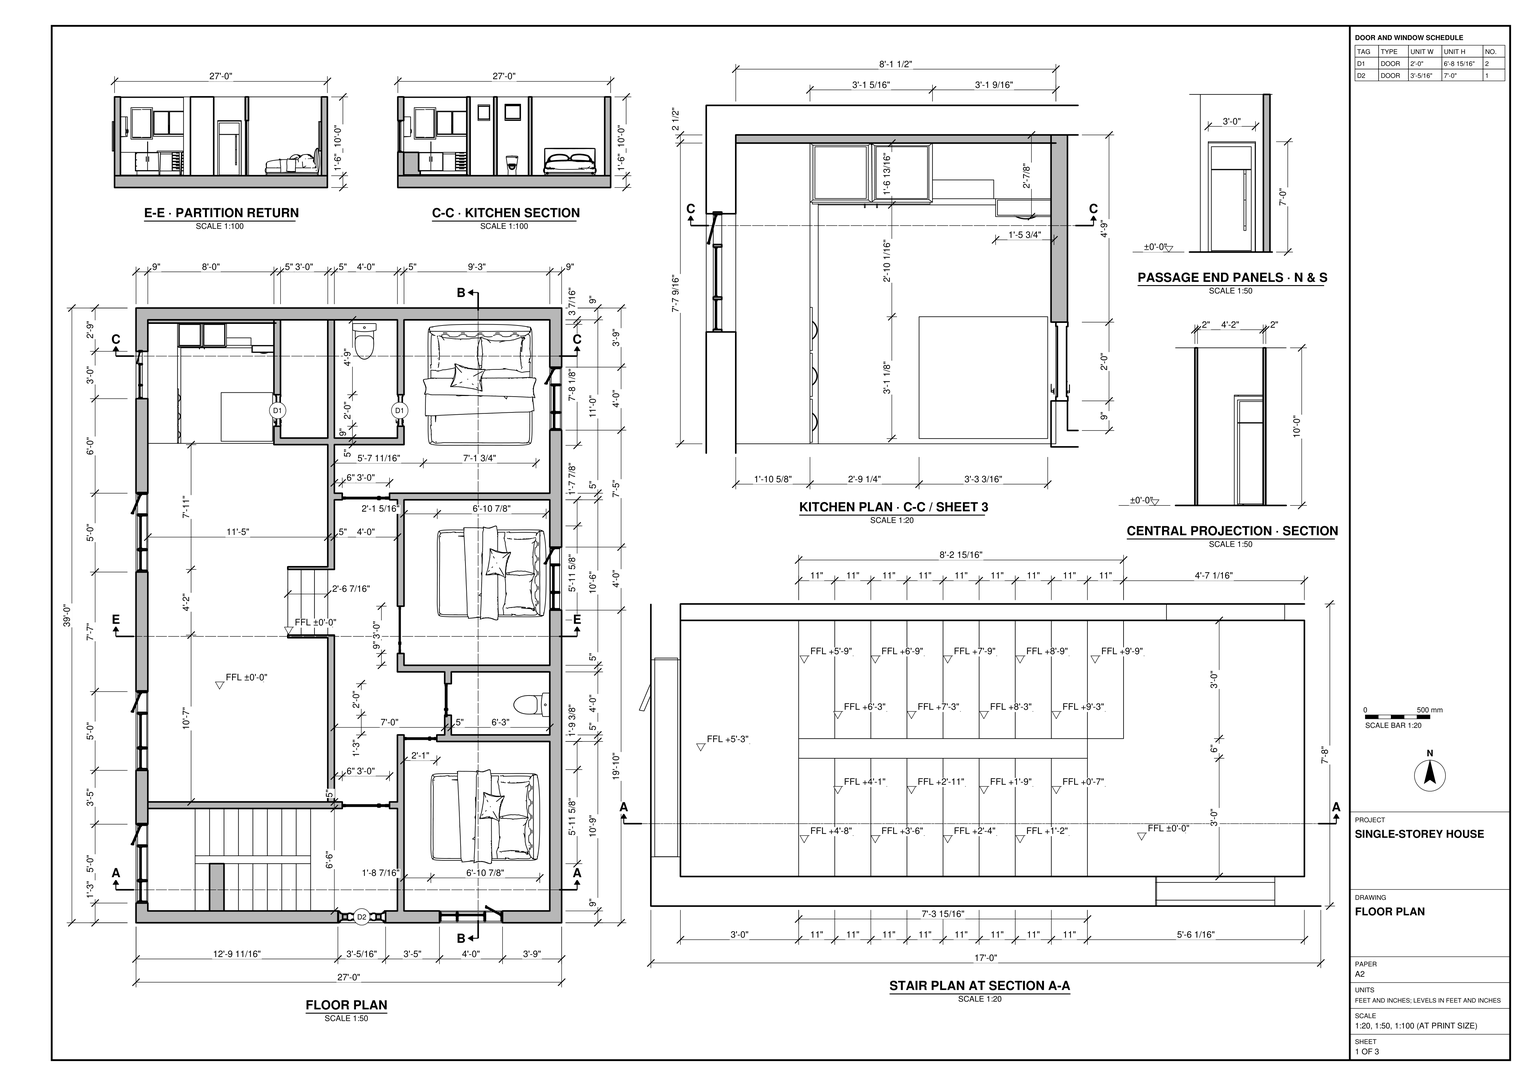
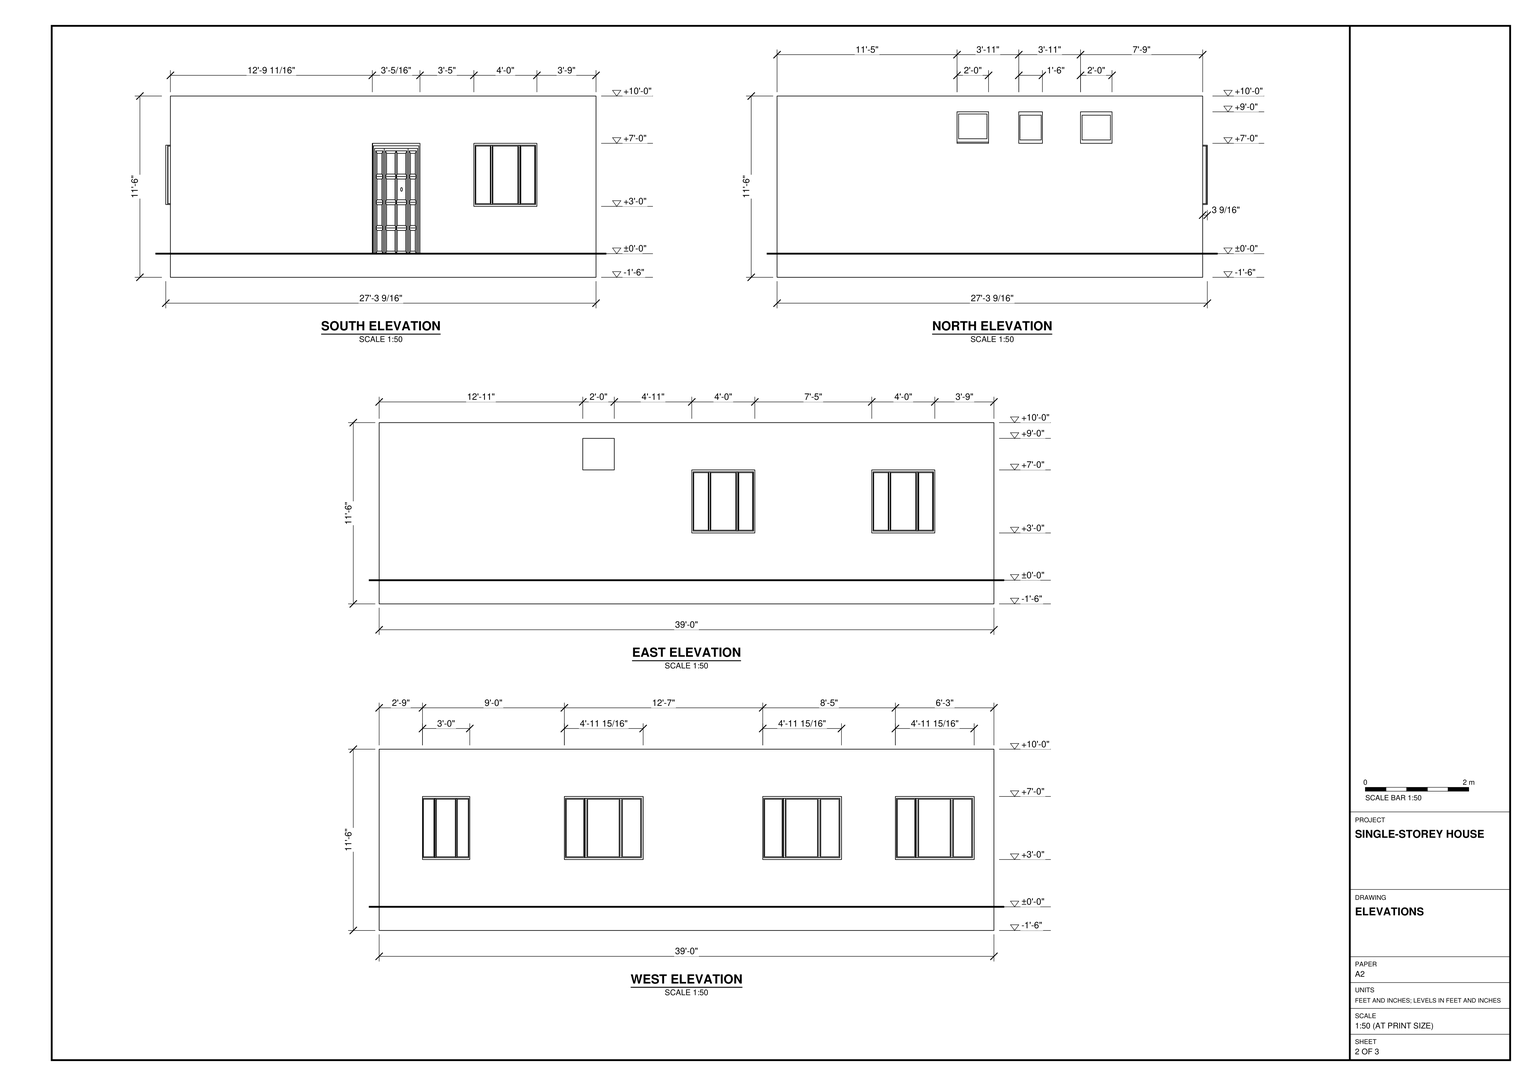
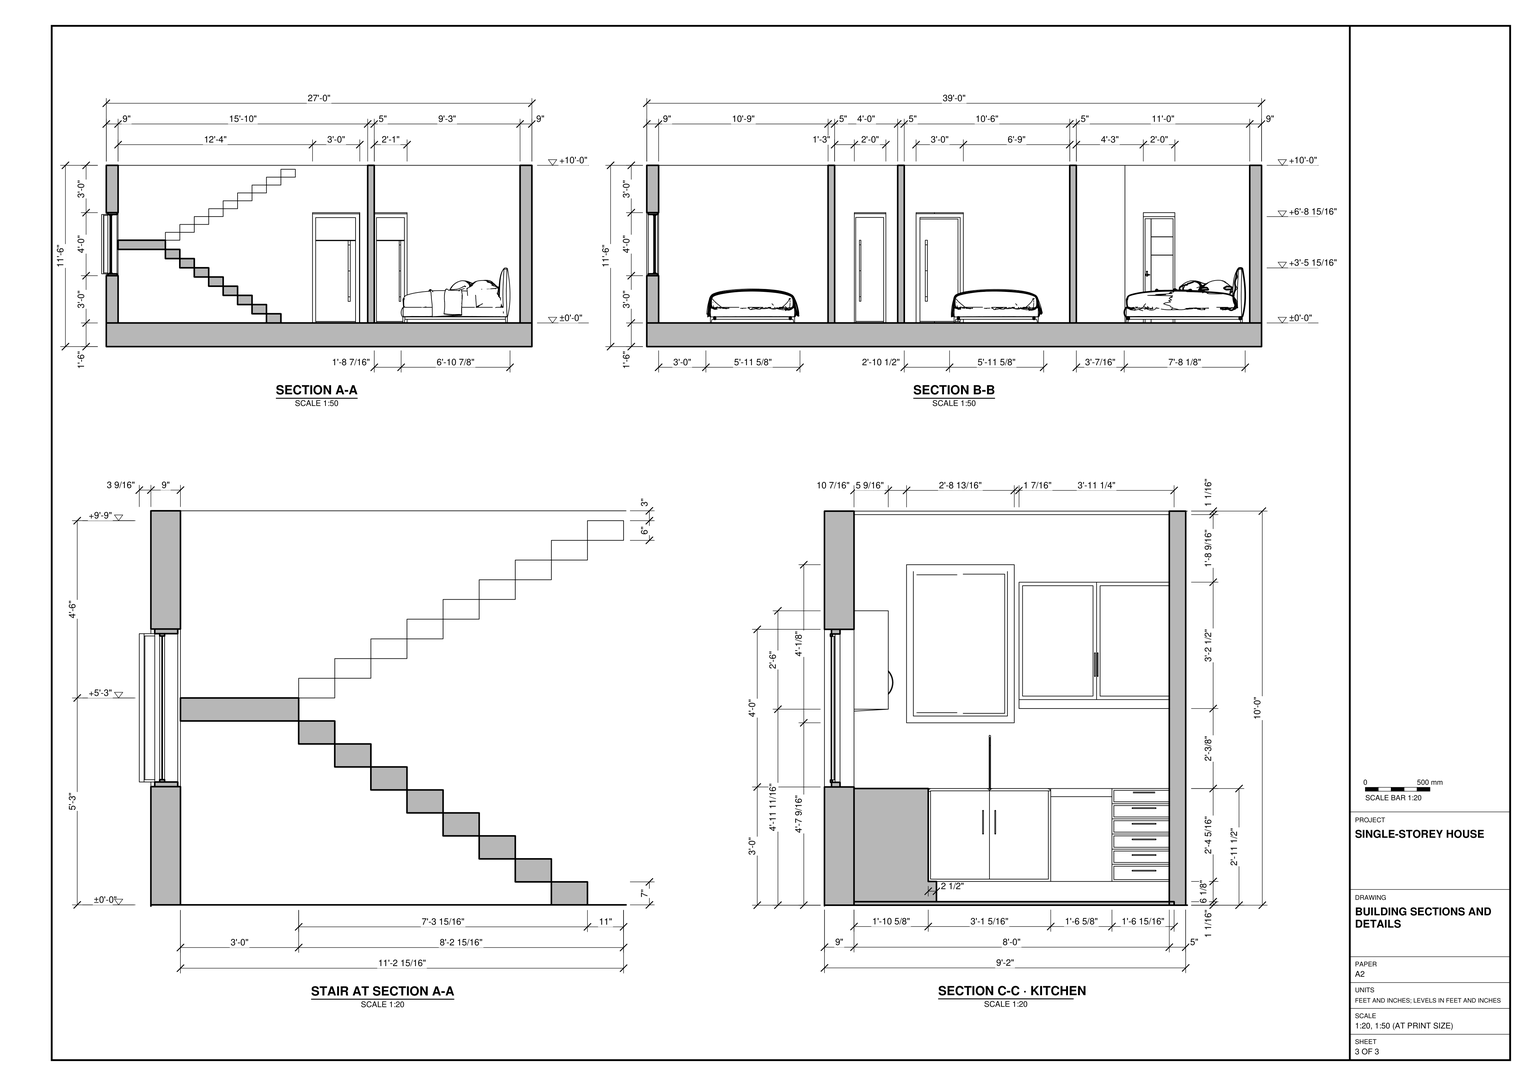
Build the single-storey house in SketchUp from task_files/diagram_01.pdf. Work in feet and inches, with the finished ground floor at ±0'-0". The overall model is 27'-3 9/16" east to west, 39'-0" north to south and 11'-6" high. The rectangular shell itself is 27'-0" wide; use the elevations to account for the projecting window frames rather than widening the walls.

Model the 1'-6" base slab, 9" exterior walls and 5" interior partitions as drawn. Place the entrance on the south side between the stair and the southeast bedroom. Follow the plan for the large open area on the west, the projecting partition return, the three bedrooms along the east side and the two toilet compartments. Fit the doors and window units to the openings shown in the plan and elevations.

Use the enlarged stair plan and section to build the two parallel flights with their shared landing against the west wall. In the northwest kitchen, follow the detailed plan and section for the worktop, base cupboards, drawer bank and wall cupboards. Size and orient the beds from the plan and building sections. Decor and loose items may be any suitable library components.

Keep shell elements separate from one another, make each furniture or joinery piece a separate group or component, and use components for repeated parts. Save one SketchUp model as output_files/single_storey_house_with_return_stair_and_kitchen.skp.

# SketchUp Ruby script. Lengths in inches.
U = 1.inch
M = Sketchup.active_model
def pt(a) = Geom::Point3d.new(a.map { |v| v * U })
def face(e, loops, mat)
  f = e.add_face(loops[0].map { |a| pt(a) })
  loops[1..].each { |l| e.add_face(l.map { |a| pt(a) }).erase! }
  f.material = f.back_material = mat if mat
  f
end
# faces: each face lists its corners as indices into pts; further lists are holes
def faces(e, pts, list, mat = nil) = list.each { |f| face(e, (f[0].is_a?(Array) ? f : [f]).map { |l| l.map { |i| pts[i] } }, mat) }
# xy, xz, yz: faces in a plane at the given z, y or x. An outline is a flat list of corners, or four numbers for a rectangle; further outlines are holes
def ring(l) = l.size == 4 ? [[l[0], l[1]], [l[2], l[1]], [l[2], l[3]], [l[0], l[3]]] : l.each_slice(2).to_a
def flat(e, list, mat, &to3) = list.each { |f| face(e, (f[0].is_a?(Array) ? f : [f]).map { |l| ring(l).map { |u, v| to3.(u, v) } }, mat) }
def xy(e, z, list, mat = nil) = flat(e, list, mat) { |x, y| [x, y, z] }
def xz(e, y, list, mat = nil) = flat(e, list, mat) { |x, z| [x, y, z] }
def yz(e, x, list, mat = nil) = flat(e, list, mat) { |y, z| [x, y, z] }
def lines(e, pts, list) = list.each { |a, b| e.add_line(pt(pts[a]), pt(pts[b])) }
# prism: a flat outline (further loops are holes) pulled along v
def prism(e, loops, v, mat = nil)
  f = face(e, loops, mat); d = Geom::Vector3d.new(v.map { |x| x * U })
  f.pushpull(f.normal.samedirection?(d) ? d.length : -d.length)
end
def box(e, o, s, mat = nil) = prism(e, [[o, [o[0] + s[0], o[1], o[2]], [o[0] + s[0], o[1] + s[1], o[2]], [o[0], o[1] + s[1], o[2]]]], [0, 0, s[2]], mat)
def at(x, y, z, deg = 0) = Geom::Transformation.translation(pt([x, y, z])) * Geom::Transformation.rotation(ORIGIN, Z_AXIS, deg.degrees)
def axes(o, x, y, z) = Geom::Transformation.new([*x, 0, *y, 0, *z, 0, *pt(o).to_a, 1])
def part(name) = M.definitions.add(name)
# library, detail: a bought-in or finely detailed component or shape, given as its bounding box
def library(name, o, s) = part(name).tap { |d| box(d.entities, o, s) }
def detail(e, o, s) = box(e.add_group.entities, o, s)
def put(e, d, t, mat = nil) = e.add_instance(d, t).tap { |i| i.material = mat if mat }
def group(e, t, mat = nil) = e.add_group.tap { |g| g.transformation = t; g.material = mat if mat }.entities
root = M.entities
M.materials.add("Doors_Windows").color = [200, 200, 200]
M.materials.add("Rectangles Running 2x1").color = [231, 231, 231]
M.materials.add("[0011_Seashell]").color = [255, 245, 238]
M.materials.add("[0130_Gainsboro]").color = [220, 220, 220]
M.materials.add("[Color_000]").color = [255, 255, 255]
M.materials.add("[Metal_Aluminum_Anodized]1").color = [202, 209, 219]
M.materials.add("[Stone_Masonry_Multi]").color = [182, 175, 164]
M.materials.add("[Stone_Sandstone_Ashlar_Light]1").color = [206, 178, 128]
M.materials.add("[Translucent Glass Blue]").color = [100, 149, 237]
M.materials["[Translucent Glass Blue]"].alpha = 0.5
M.materials.add("[Translucent_Glass_Safety]").color = [204, 235, 244]
M.materials["[Translucent_Glass_Safety]"].alpha = 0.5
M.materials.add("[Wood Cherry Original]").color = [152, 86, 42]
M.materials.add("[Wood_Bamboo_Medium]").color = [177, 105, 43]
M.materials.add("[Wood_Floor_Parquet]").color = [145, 89, 39]
M.materials.add("[Wood_OSB]").color = [240, 195, 122]
c1 = part("bod vindu")
g1 = group(c1.entities,at(0,-46.85,0),"[Translucent Glass Blue]")
yz(g1,0.94,[[2.36,2.36,44.49,19.65]],"[Translucent Glass Blue]")
# 2 loose lines left out
g2 = group(g1,at(0,46.85,0,-90),"[Color_000]")
xy(g2,0,[[0,0,46.85,3.9375]])
xy(g2,1.57,[[1.57,0,45.28,0.55]])
xy(g2,2.36,[[2.36,0.55,44.49,3.9375]])
xy(g2,19.65,[[2.36,0.55,4.29,3.9375],[4.29,0.55,44.49,3.9375]])
xy(g2,20.43,[[1.57,0,45.28,0.55]])
xy(g2,22.01,[[0,0,46.85,3.9375]])
xz(g2,0,[[[0,0,46.85,22.01],[1.57,1.57,45.28,20.43]]])
xz(g2,0.55,[[1.57,1.57,45.28,2.36],[1.57,2.36,2.36,2.36,2.36,19.65,44.49,19.65,44.49,2.36,45.28,2.36,45.28,20.43,1.57,20.43]])
xz(g2,3.9375,[[[0,0,46.85,22.01],[2.36,2.36,44.49,19.65]]])
yz(g2,0,[[0,0,3.9375,22.01]])
yz(g2,1.57,[[0,1.57,0.55,2.36,0.55,20.43,0,20.43]])
yz(g2,2.36,[[0.55,2.36,3.9375,19.65]])
yz(g2,44.49,[[0.55,2.36,3.9375,19.65]])
yz(g2,45.28,[[0,1.57,0,20.43,0.55,20.43,0.55,2.36]])
yz(g2,46.85,[[0,0,3.9375,22.01]])
p = [[45.28,0,1.57],[1.57,0,1.57],[1.57,0.55,2.36],[2.36,0.55,2.36],[44.49,0.55,2.36],[45.28,0.55,2.36]]
faces(g2,p,[[0,1,2,3,4,5]])
c2 = library("Door",[0,0,0],[79.98,10,87.99])
c3 = library("porta de madeira",[3.7,-4.82,1.36],[53.55,7.65,83.26])
c4 = library("Door\#1",[0,0,0],[31.5,7.64,86.61])
c5 = library("CS300DRT",[0,0,0],[27.18,17.85,30.31])
c6 = part("Group\#36")
box(c6.entities,[-2,0,0],[2,7,64])
c7 = part("Group\#6")
xy(c7.entities,0,[[0,-7,96,0]])
xy(c7.entities,2,[[2,-7,94,0]])
xy(c7.entities,66,[[2,-7,94,0]])
xy(c7.entities,68,[[0,-7,96,0]])
xz(c7.entities,-7,[[[0,0,96,68],[2,2,94,66]]])
xz(c7.entities,0,[[[0,0,96,68],[2,2,94,66]]])
yz(c7.entities,0,[[-7,0,0,68]])
yz(c7.entities,2,[[-7,2,0,66]])
yz(c7.entities,94,[[-7,2,0,66]])
yz(c7.entities,96,[[-7,0,0,68]])
put(c7.entities,c6,at(70,-7,2))
put(c7.entities,c6,at(28,-7,2))
g3 = group(c7.entities,at(70.82,4.71,2,-15),"[Translucent Glass Blue]")
xy(g3,0,[[0,-1.5,24,0]],"Doors_Windows")
xy(g3,1,[[1,-1.5,23,-0.75],[1,-0.75,23,0]],"Doors_Windows")
xy(g3,63,[[1,-1.5,23,-0.75],[1,-0.75,23,0]],"Doors_Windows")
xy(g3,64,[[0,-1.5,24,0]],"Doors_Windows")
xz(g3,-1.5,[[[0,0,24,64],[1,1,23,63]]],"Doors_Windows")
xz(g3,-0.75,[[1,1,23,63]],"[Translucent Glass Blue]")
xz(g3,0,[[[0,0,24,64],[1,1,23,63]]],"Doors_Windows")
yz(g3,0,[[-1.5,0,0,64]],"Doors_Windows")
yz(g3,1,[[-1.5,1,-0.75,63],[-0.75,1,0,63]],"Doors_Windows")
yz(g3,23,[[-1.5,1,-0.75,63],[-0.75,1,0,63]],"Doors_Windows")
yz(g3,24,[[-1.5,0,0,64]],"Doors_Windows")
g4 = group(c7.entities,at(2,-1.5,2))
xy(g4,0,[[0,-1.5,24,0]],"[Translucent Glass Blue]")
xy(g4,1,[[1,-1.5,23,-0.75],[1,-0.75,23,0]],"[Translucent Glass Blue]")
xy(g4,63,[[1,-1.5,23,-0.75],[1,-0.75,23,0]],"[Translucent Glass Blue]")
xy(g4,64,[[0,-1.5,24,0]],"[Translucent Glass Blue]")
xz(g4,-1.5,[[[0,0,24,64],[1,1,23,63]]],"[Translucent Glass Blue]")
xz(g4,-0.75,[[1,1,23,63]],"[Translucent Glass Blue]")
xz(g4,0,[[[0,0,24,64],[1,1,23,63]]],"[Translucent Glass Blue]")
yz(g4,0,[[-1.5,0,0,64]],"[Translucent Glass Blue]")
yz(g4,1,[[-1.5,1,-0.75,63],[-0.75,1,0,63]],"[Translucent Glass Blue]")
yz(g4,23,[[-1.5,1,-0.75,63],[-0.75,1,0,63]],"[Translucent Glass Blue]")
yz(g4,24,[[-1.5,0,0,64]],"[Translucent Glass Blue]")
g5 = group(c7.entities,at(28,-1.5,2),"[Translucent Glass Blue]")
xy(g5,0,[[0,-1.5,40,0]],"Doors_Windows")
xy(g5,1,[[1,-1.5,39,-0.75],[1,-0.75,39,0]],"Doors_Windows")
xy(g5,63,[[1,-1.5,39,-0.75],[1,-0.75,39,0]],"Doors_Windows")
xy(g5,64,[[0,-1.5,40,0]],"Doors_Windows")
xz(g5,-1.5,[[[0,0,40,64],[1,1,39,63]]],"Doors_Windows")
xz(g5,-0.75,[[1,1,39,63]],"[Translucent Glass Blue]")
xz(g5,0,[[[0,0,40,64],[1,1,39,63]]],"Doors_Windows")
yz(g5,0,[[-1.5,0,0,64]],"Doors_Windows")
yz(g5,1,[[-1.5,1,-0.75,63],[-0.75,1,0,63]],"Doors_Windows")
yz(g5,39,[[-1.5,1,-0.75,63],[-0.75,1,0,63]],"Doors_Windows")
yz(g5,40,[[-1.5,0,0,64]],"Doors_Windows")
c8 = part("Group\#84")
box(c8.entities,[0,0,0],[10.99,36,7])
c9 = part("Group\#85")
box(c9.entities,[0,0,0],[10.99,36,6])
c10 = library("Group10",[-94.75,-3.97,0],[199.87,106.11,39.4375])
c11 = library("mesh-258",[-96.03,-121.28,21.97],[201.42,163.89,40.48])
c12 = library("Group14",[-46.92,-34.29,0],[94.87,68.58,31.875])
c13 = library("Group16",[-47.82,-34.55,0],[96.75,69.58,33.34])
c14 = library("Group18",[-33.62,-26.58,0],[67.24,53.16,20.44])
c15 = library("Group20",[-0.01,-0.01,0.02],[107.76,124.16,6.31])
c16 = library("mesh-263",[-97.08,-118.58,12.75],[201.41,233.93,94.93])
c17 = library("mesh-264",[-106.11,-80.86,12.52],[217.88,74.95,54.44])
c18 = part("Group9")
put(c18.entities,c10,axes([-2.83,3.64,23.125],[0.96274,0,0],[0,0.96274,0],[0,0,0.96274]))
g6 = group(c18.entities,at(-2.83,3.64,23.41))
put(g6,c11,axes([0,0,-21.09],[0.96274,0,0],[0,0.96274,0],[0,0,0.96274]))
put(c18.entities,c12,at(49.15,58.47,50.125))
put(c18.entities,c13,at(-47.3,60.89,49.06))
put(c18.entities,c14,at(-22.74,14.21,61.08))
put(c18.entities,c15,axes([-96.54,-113.26,0],[1.80992,0,0],[0,1.80992,0],[0,0,1.80992]))
g7 = group(c18.entities,at(-2.83,1.61,11.33))
put(g7,c16,at(0,0,-12.75))
g8 = group(c18.entities,at(-2.83,20.36,11.1))
put(g8,c17,at(0,0,-12.52))
c19 = library("Group\#91",[0,0,0],[8.9,40.12,1.52])
c20 = part("Group\#92")
xy(c20.entities,0,[[0,0,117.79,26.26]])
c21 = part("Group\#93")
box(c21.entities,[0,0,0],[32.88,158.35,2.28])
c22 = part("Tapered column")
xy(c22.entities,0,[[0,0,24.46,29.02]])
xy(c22.entities,262.42,[[7.21,8.5625,17.24,20.46]])
p = [[7.21,8.5625,262.42],[7.21,20.46,262.42],[0,29.02,0],[0,0,0],[24.46,0,0],[17.24,8.5625,262.42],
  [24.46,29.02,0],[17.24,20.46,262.42]]
faces(c22.entities,p,[[0,1,2,3],[4,5,0,3],[4,6,7,5],[2,1,7,6]])
xy(root,1.07,[[12.54,364.95,37.64,364.95,37.64,437.69,110.01,437.69,110.01,456.52,12.54,456.52]])
xy(root,7.22,[[35.13,364.95,37.64,438.5],[37.64,437.69,37.64,438.5,72.43,438.5,72.43,439.58,110.01,439.58,110.01,437.69]],"[Wood_Bamboo_Medium]")
xy(root,7.79,[[35.13,365.375,35.85,378.5],[35.13,379.36,35.85,392.49],[35.13,393.35,35.85,406.47],[91.66,439.04,109.43,439.58]])
xy(root,7.93,[[35.85,437.96,37.64,438.5],[37.64,437.96,71.71,438.5]])
xy(root,11.87,[[91.66,439.04,109.43,439.58]],"[Wood_Bamboo_Medium]")
xy(root,13,[[91.66,439.04,109.43,439.58]])
xy(root,16.49,[[35.13,365.375,35.85,378.5],[35.13,379.36,35.85,392.49],[35.13,393.35,35.85,406.47],[91.66,439.04,109.43,439.58]],"[Wood_Bamboo_Medium]")
xy(root,17.62,[[35.13,365.375,35.85,378.5],[35.13,379.36,35.85,392.49],[35.13,393.35,35.85,406.47],[91.66,439.04,109.43,439.58]])
xy(root,21.1,[[91.66,439.04,109.43,439.58]],"[Wood_Bamboo_Medium]")
xy(root,22.24,[[91.66,439.04,109.43,439.58]])
xy(root,25.72,[[35.13,365.375,35.85,378.5],[35.13,379.36,35.85,392.49],[35.13,393.35,35.85,406.47],[91.66,439.04,109.43,439.58]],"[Wood_Bamboo_Medium]")
xy(root,26.86,[[35.13,365.375,35.85,378.5],[35.13,379.36,35.85,392.49],[91.66,439.04,109.43,439.58]])
xy(root,26.86,[[35.13,393.35,35.85,406.47]],"[Wood_Bamboo_Medium]")
xy(root,30.34,[[91.66,439.04,109.43,439.58]],"[Wood_Bamboo_Medium]")
xy(root,31.48,[[91.66,434.12,109.43,439.58]],"[Wood_Bamboo_Medium]")
xy(root,32.6875,[[36.64,439.63,52.28,455.39],[55.29,439.63,70.93,455.39]],"[Metal_Aluminum_Anodized]1")
xy(root,33.06,[[72.43,439.58,91.08,445.3]],"Rectangles Running 2x1")
xy(root,33.24,[[92.23,434.55,108.86,439.15]],"[Wood_Bamboo_Medium]")
xy(root,34.82,[[35.85,437.96,71.71,438.5]],"[Wood_Bamboo_Medium]")
xy(root,34.96,[[35.13,365.375,35.85,378.5],[35.13,379.36,35.85,392.49],[35.13,393.35,35.85,406.47],[[91.66,434.12,109.43,439.58],[92.23,434.55,108.86,439.15]]],"[Wood_Bamboo_Medium]")
xy(root,35.53,[[12.54,364.95,35.13,456.52],[91.08,439.58,110.01,439.58,110.01,456.52,72.43,456.52,72.43,445.3,91.08,445.3]],"Rectangles Running 2x1")
xy(root,35.53,[[[36.03,439.17,52.89,455.85],[36.64,439.63,52.28,455.39]],[[54.87,439.32,71.34,455.7],[55.29,439.63,70.93,455.39]]],"[Metal_Aluminum_Anodized]1")
xy(root,55.54,[[28.53,456.52,61.33,459]],"[0011_Seashell]")
xy(root,59.67,[[12.54,364.95,21.21,380.1],[12.54,380.1,20.03,395.21]],"[0130_Gainsboro]")
xy(root,59.88,[[62.78,450.85,110.01,456.52]],"[Wood_Floor_Parquet]")
xy(root,61.48,[[20.5,364.95,21.21,380.1],[18.13,380.1,20.03,395.21]],"[0130_Gainsboro]")
xy(root,63.67,[[63.86,450.85,85.32,455.72],[87.47,450.85,108.93,455.72]],"[Wood_Floor_Parquet]")
xy(root,65.32,[[12.54,425.35,18.53,425.73]])
xy(root,65.32,[[12.54,404.09,18.53,404.5]],"[Wood_Bamboo_Medium]")
xy(root,74.57,[[63.86,452.14,85.32,455.72]],"[Wood_Floor_Parquet]")
xy(root,84.03,[[12.54,404.09,18.53,404.5]],"[Wood_Bamboo_Medium]")
xy(root,89.65,[[12.54,364.95,20.5,380.1],[12.54,380.1,18.13,395.21],[12.54,432.6,22.97,456.52]],"[0130_Gainsboro]")
xy(root,97.29,[[63.86,450.85,85.32,455.72],[87.47,450.85,108.93,455.72]],"[Wood_Floor_Parquet]")
xy(root,98.35,[[62.78,450.85,110.01,456.52]],"[Wood_Floor_Parquet]")
xy(root,103.68,[[28.53,456.52,61.33,459]],"[0011_Seashell]")
xz(root,364.95,[[12.54,59.67,12.54,89.65,20.5,89.65,20.5,61.48,21.21,61.48,21.21,59.67]],"[0130_Gainsboro]")
xz(root,364.95,[[12.54,1.07,12.54,35.53,35.13,35.53,35.13,7.22,37.64,7.22,37.64,1.07]],"[Wood_Bamboo_Medium]")
xz(root,365.375,[[35.13,7.79,35.85,16.49],[35.13,17.62,35.85,25.72],[35.13,26.86,35.85,34.96]],"[Wood_Bamboo_Medium]")
xz(root,378.5,[[35.13,7.79,35.85,16.49],[35.13,17.62,35.85,25.72],[35.13,26.86,35.85,34.96]],"[Wood_Bamboo_Medium]")
xz(root,379.36,[[35.13,7.79,35.85,16.49],[35.13,17.62,35.85,25.72],[35.13,26.86,35.85,34.96]],"[Wood_Bamboo_Medium]")
xz(root,380.1,[[12.54,59.67,20.03,59.67,20.03,61.48,18.13,61.48,18.13,89.65,12.54,89.65]])
xz(root,380.1,[[20.03,59.67,21.21,59.67,21.21,61.48,20.5,61.48,20.5,89.65,18.13,89.65,18.13,61.48,20.03,61.48]],"[0130_Gainsboro]")
xz(root,392.49,[[35.13,7.79,35.85,16.49],[35.13,17.62,35.85,25.72],[35.13,26.86,35.85,34.96]],"[Wood_Bamboo_Medium]")
xz(root,393.35,[[35.13,7.79,35.85,16.49],[35.13,17.62,35.85,25.72],[35.13,26.86,35.85,34.96]],"[Wood_Bamboo_Medium]")
xz(root,395.21,[[12.54,59.67,20.03,59.67,20.03,61.48,18.13,61.48,18.13,89.65,12.54,89.65]],"[0130_Gainsboro]")
xz(root,404.09,[[12.54,65.32,18.53,84.03]],"[Wood_Bamboo_Medium]")
xz(root,404.5,[[12.54,65.32,18.53,84.03]],"[Wood_Bamboo_Medium]")
xz(root,406.47,[[35.13,7.79,35.85,16.49],[35.13,17.62,35.85,25.72],[35.13,26.86,35.85,34.96]],"[Wood_Bamboo_Medium]")
xz(root,425.35,[[12.54,65.32,18.53,65.32,18.53,84.03,12.54,83.89]],"[Wood_Bamboo_Medium]")
xz(root,425.73,[[12.54,65.32,12.54,83.89,18.53,84.03,18.53,65.32]],"[Wood_Bamboo_Medium]")
xz(root,432.6,[[12.54,59.67,22.97,89.65]],"[0130_Gainsboro]")
xz(root,434.12,[[91.66,31.48,109.43,34.96]],"[Wood_Bamboo_Medium]")
xz(root,434.55,[[92.23,33.24,108.86,34.96]])
xz(root,437.69,[[37.64,1.07,110.01,7.22]],"[Wood_Bamboo_Medium]")
xz(root,437.96,[[35.85,7.93,53.78,34.82],[53.78,7.93,71.71,34.82]],"[Wood_Bamboo_Medium]")
xz(root,438.5,[[35.13,7.22,72.43,7.22,72.43,34.82,71.71,34.82,71.71,7.93,35.85,7.93,35.85,34.64,35.13,34.64]],"[Wood_OSB]")
xz(root,439.04,[[91.66,7.79,109.43,11.87],[91.66,13,109.43,16.49],[91.66,17.62,109.43,21.1],[91.66,22.24,109.43,25.72],[91.66,26.86,109.43,30.34]],"[Wood_Bamboo_Medium]")
xz(root,439.15,[[92.23,33.24,108.86,34.96]],"[Wood_Bamboo_Medium]")
xz(root,439.58,[[72.43,7.22,91.08,33.06]],"[Wood_Bamboo_Medium]")
xz(root,439.58,[[[91.08,7.22,110.01,12.43],[91.66,7.79,109.43,11.87]],[[91.08,12.43,110.01,17.05],[91.66,13,109.43,16.49]],[[91.08,17.05,110.01,21.67],[91.66,17.62,109.43,21.1]],[[91.08,21.67,110.01,26.29],[91.66,22.24,109.43,25.72]],[[91.08,26.29,110.01,30.91],[91.66,26.86,109.43,30.34]],
  [[91.08,30.91,110.01,35.53],[91.66,31.48,109.43,34.96]]],"[Wood_OSB]")
xz(root,439.63,[[36.64,32.6875,52.28,35.53],[55.29,32.6875,70.93,35.53]])
xz(root,445.3,[[72.43,33.06,91.08,35.53]],"Rectangles Running 2x1")
xz(root,450.85,[[63.86,63.67,85.32,97.29],[87.47,63.67,108.93,97.29]],"[Translucent_Glass_Safety]")
xz(root,450.85,[[[62.78,62.61,86.39,98.35],[63.86,63.67,85.32,97.29]],[[86.39,62.61,110.01,98.35],[87.47,63.67,108.93,97.29]]],"[Wood_Floor_Parquet]")
xz(root,450.85,[[62.78,59.88,110.01,62.61]],"[Wood_OSB]")
xz(root,455.39,[[36.64,32.6875,52.28,35.53],[55.29,32.6875,70.93,35.53]],"[Metal_Aluminum_Anodized]1")
xz(root,455.72,[[63.86,63.67,85.32,74.57],[87.47,63.67,108.93,97.29],[63.86,74.57,85.32,89.1],[63.86,89.1,85.32,97.29]],"[Wood_Floor_Parquet]")
xz(root,456.52,[[62.78,59.88,110.01,98.35]])
xz(root,456.52,[[12.54,1.07,110.01,1.07,110.01,35.53,72.43,35.53,72.43,34.82,53.78,34.82,53.78,34.64,35.13,34.64,35.13,35.53,12.54,35.53],[35.13,34.64,53.78,35.53],[53.78,34.82,72.43,35.53]],"[Metal_Aluminum_Anodized]1")
xz(root,456.52,[[[12.54,35.53,110.01,35.53,110.01,59.88,62.78,59.88,62.78,98.35,110.01,98.35,110.01,118.93,12.54,118.93,12.54,89.65,22.97,89.65,22.97,59.67,12.54,59.09],[28.53,55.54,61.33,103.68]],[12.54,59.09,22.97,59.67,22.97,89.65,12.54,89.65]],"[Stone_Sandstone_Ashlar_Light]1")
yz(root,12.54,[[364.95,1.07,456.52,35.53],[364.95,59.67,380.1,89.65],[380.1,59.67,395.21,89.65]])
yz(root,12.54,[[456.52,59.09,456.52,89.65,432.6,89.65,432.6,59.67],[404.09,65.32,404.5,84.03],[425.35,65.32,425.73,83.89]],"[Stone_Sandstone_Ashlar_Light]1")
yz(root,18.13,[[380.1,61.48,395.21,89.65]],"[0130_Gainsboro]")
yz(root,18.53,[[404.09,65.32,404.5,84.03],[425.35,65.32,425.73,84.03]],"[Wood_Bamboo_Medium]")
yz(root,20.03,[[380.1,59.67,395.21,61.48]],"[Wood_OSB]")
yz(root,20.5,[[364.95,61.48,380.1,89.65]],"[0130_Gainsboro]")
yz(root,21.21,[[364.95,59.67,380.1,61.48]],"[Wood_OSB]")
yz(root,22.97,[[432.6,61.71,456.52,89.65]],"[0130_Gainsboro]")
yz(root,22.97,[[432.6,59.67,456.52,61.71]],"[Wood_OSB]")
yz(root,28.53,[[456.52,55.54,459,103.68]],"[0011_Seashell]")
yz(root,35.13,[[438.5,34.64,456.52,35.53]])
yz(root,35.13,[[406.9,7.22,420.89,35.53],[420.89,7.22,438.5,35.53]],"[Wood_Bamboo_Medium]")
yz(root,35.13,[[[364.95,7.22,378.93,17.05],[365.375,7.79,378.5,16.49]],[[378.93,7.22,392.92,17.05],[379.36,7.79,392.49,16.49]],[[392.92,7.22,406.9,17.05],[393.35,7.79,406.47,16.49]],[[364.95,17.05,378.93,26.29],[365.375,17.62,378.5,25.72]],[[378.93,17.05,392.92,26.29],[379.36,17.62,392.49,25.72]],
  [[392.92,17.05,406.9,26.29],[393.35,17.62,406.47,25.72]],[[364.95,26.29,378.93,35.53],[365.375,26.86,378.5,34.96]],[[378.93,26.29,392.92,35.53],[379.36,26.86,392.49,34.96]],[[392.92,26.29,406.9,35.53],[393.35,26.86,406.47,34.96]]],"[Wood_OSB]")
yz(root,35.85,[[437.96,7.93,438.5,34.82]])
yz(root,35.85,[[365.375,7.79,378.5,16.49],[379.36,7.79,392.49,16.49],[393.35,7.79,406.47,16.49],[365.375,17.62,378.5,25.72],[379.36,17.62,392.49,25.72],
  [393.35,17.62,406.47,25.72],[365.375,26.86,378.5,34.96],[379.36,26.86,392.49,34.96],[393.35,26.86,406.47,34.96]],"[Wood_Bamboo_Medium]")
yz(root,36.64,[[439.63,32.6875,455.39,35.53]],"[Metal_Aluminum_Anodized]1")
yz(root,37.64,[[364.95,1.07,437.69,7.22]],"[Wood_Bamboo_Medium]")
yz(root,52.28,[[439.63,32.6875,455.39,35.53]],"[Metal_Aluminum_Anodized]1")
yz(root,53.78,[[438.5,34.64,456.52,34.82]])
yz(root,55.29,[[439.63,32.6875,455.39,35.53]],"[Metal_Aluminum_Anodized]1")
yz(root,61.33,[[456.52,55.54,459,103.68]],"[0011_Seashell]")
yz(root,62.78,[[450.85,59.88,456.52,98.35]],"[Wood_Floor_Parquet]")
yz(root,63.86,[[450.85,63.67,455.72,97.29]],"[Wood_Floor_Parquet]")
yz(root,70.93,[[439.63,32.6875,455.39,35.53]],"[Metal_Aluminum_Anodized]1")
yz(root,71.71,[[437.96,7.93,438.5,34.82]],"[Wood_Bamboo_Medium]")
yz(root,72.43,[[438.5,7.22,439.58,7.22,439.58,33.06,445.3,33.06,445.3,34.82,438.5,34.82]],"[Wood_Bamboo_Medium]")
yz(root,85.32,[[450.85,63.67,455.72,97.29]],"[Wood_Floor_Parquet]")
yz(root,87.47,[[450.85,63.67,455.72,97.29]],"[Wood_Floor_Parquet]")
yz(root,91.08,[[439.58,33.06,445.3,35.53]],"[Metal_Aluminum_Anodized]1")
yz(root,91.66,[[439.04,7.79,439.58,11.87],[439.04,13,439.58,16.49],[439.04,17.62,439.58,21.1],[439.04,22.24,439.58,25.72],[439.04,26.86,439.58,30.34],
  [434.12,31.48,439.58,34.96]],"[Wood_Bamboo_Medium]")
yz(root,92.23,[[434.55,33.24,439.15,34.96]],"[Wood_Bamboo_Medium]")
yz(root,108.86,[[434.55,33.24,439.15,34.96]],"[Wood_Bamboo_Medium]")
yz(root,108.93,[[450.85,63.67,455.72,97.29]],"[Wood_Floor_Parquet]")
yz(root,109.43,[[439.04,7.79,439.58,11.87],[439.04,13,439.58,16.49],[439.04,17.62,439.58,21.1],[439.04,22.24,439.58,25.72],[439.04,26.86,439.58,30.34],
  [434.12,31.48,439.58,34.96]],"[Wood_Bamboo_Medium]")
yz(root,110.01,[[437.69,1.07,456.52,1.07,456.52,35.53,439.58,35.53,439.58,7.22,437.69,7.22]],"[Wood_Bamboo_Medium]")
yz(root,110.01,[[450.85,59.88,456.52,98.35]],"[Wood_Floor_Parquet]")
# 42 loose lines left out
p = [[35.13,438.5,34.64],[35.14,438.51,34.76],[35.14,456.51,34.76],[35.13,456.52,34.64],[35.85,438.5,34.64],[36.03,438.5,34.64],
  [53.78,438.5,34.64],[53.77,438.51,34.76],[36.03,438.51,34.76],[53.78,456.52,34.64],[53.77,456.51,34.76],[35.16,438.52,34.87],
  [35.16,456.5,34.87],[53.75,438.52,34.87],[36.03,438.52,34.87],[53.78,438.5,34.82],[53.83,438.54,34.92],[53.83,456.48,34.92],
  [53.78,456.52,34.82],[53.75,456.5,34.87],[72.43,438.5,34.82],[72.38,438.54,34.92],[54.87,438.54,34.92],[54.87,438.5,34.82],
  [71.71,438.5,34.82],[72.43,445.3,34.82],[72.43,456.52,34.82],[72.38,456.48,34.92],[72.38,445.3,34.92],[35.2,438.55,34.98],
  [35.2,456.47,34.98],[53.71,438.55,34.98],[36.03,438.55,34.98],[53.71,456.47,34.98],[53.89,438.58,35.02],[53.89,456.4375,35.02],
  [72.32,438.58,35.02],[54.87,438.58,35.02],[72.32,456.4375,35.02],[72.32,445.3,35.02],[35.25,438.59,35.08],[35.25,456.43,35.08],
  [53.66,438.59,35.08],[36.03,438.59,35.08],[53.66,456.43,35.08],[53.96,438.64,35.11],[53.96,456.39,35.11],[72.25,438.64,35.11],
  [54.87,438.64,35.11],[72.25,456.39,35.11],[72.25,445.3,35.11],[53.6,438.64,35.18],[36.03,438.64,35.18],[35.32,438.64,35.18],
  [35.32,456.38,35.18],[53.6,456.38,35.18],[72.17,438.69,35.19],[54.87,438.69,35.19],[54.04,438.69,35.19],[72.17,456.33,35.19],
  [72.17,445.3,35.19],[53.9,456.33,35.19],[53.52,438.7,35.27],[36.03,438.7,35.27],[35.39,438.7,35.27],[35.39,456.32,35.27],
  [53.52,456.32,35.27],[54.125,438.76,35.27],[72.09,438.76,35.27],[54.87,438.76,35.27],[72.09,456.26,35.27],[72.09,445.3,35.27],
  [54.125,456.26,35.27],[53.43,438.76,35.34],[36.03,438.76,35.34],[35.48,438.76,35.34],[35.48,456.26,35.34],[53.43,456.26,35.34],
  [53.33,438.84,35.41],[36.03,438.84,35.41],[35.58,438.84,35.41],[35.58,456.18,35.41],[53.33,456.18,35.41],[54.22,438.83,35.33],
  [54.22,456.19,35.33],[72,438.83,35.33],[54.87,438.83,35.33],[54.32,438.9,35.39],[54.32,456.12,35.39],[71.9,438.9,35.39],
  [54.87,438.9,35.39],[72,445.3,35.33],[72,456.19,35.33],[71.9,456.12,35.39],[71.9,445.3,35.39],[53.23,438.92,35.46],
  [36.03,438.92,35.46],[35.68,438.92,35.46],[35.68,456.11,35.46],[53.23,456.11,35.46],[54.42,438.98,35.44],[54.42,456.04,35.44],
  [71.79,438.98,35.44],[54.87,438.98,35.44],[71.79,456.04,35.44],[71.79,445.3,35.44],[54.53,439.0625,35.48],[54.53,455.96,35.48],
  [71.68,439.0625,35.48],[54.87,439.0625,35.48],[71.68,455.96,35.48],[71.68,445.3,35.48],[53.12,439,35.5],[36.03,439,35.5],
  [35.8,439,35.5],[35.8,456.02,35.5],[53.12,456.02,35.5],[53,439.09,35.52],[36.03,439.09,35.52],[35.91,439.09,35.52],
  [35.91,455.9375,35.52],[53,455.9375,35.52],[52.89,439.17,35.53],[36.03,439.17,35.53],[36.03,455.85,35.53],[52.89,455.85,35.53],
  [54.64,439.15,35.51],[54.64,455.875,35.51],[71.57,439.15,35.51],[54.87,439.15,35.51],[54.75,439.23,35.52],[54.75,455.79,35.52],
  [71.46,439.23,35.52],[54.87,439.23,35.52],[71.57,445.3,35.51],[71.57,455.875,35.51],[71.46,455.79,35.52],[71.46,445.3,35.52],
  [54.87,439.32,35.53],[54.87,455.7,35.53],[71.34,439.32,35.53],[71.34,455.7,35.53],[71.34,445.3,35.53],[22.97,432.6,59.67],
  [12.54,456.52,59.09],[12.54,432.6,59.67],[22.97,456.52,59.67],[18.53,425.73,84.03],[12.54,425.73,83.89],[12.54,425.35,83.89],
  [18.53,425.35,84.03]]
faces(root,p,[[0,1,2,3],[4,5,6,7,8,1,0],[9,10,7,6],[3,2,10,9],[1,11,12,2],[1,8,7,13,14,11],[15,16,17,18],[10,19,13,7],
  [20,21,22,16,15,23,24],[20,25,26,27,28,21],[2,12,19,10],[18,17,27,26],[11,29,30,12],[11,14,13,31,32,29],[19,33,31,13],[16,34,35,17],
  [21,36,37,34,16,22],[21,28,27,38,39,36],[17,35,38,27],[12,30,33,19],[29,40,41,30],[29,32,31,42,43,40],[33,44,42,31],[34,45,46,35],
  [36,47,48,45,34,37],[36,39,38,49,50,47],[30,41,44,33],[35,46,49,38],[40,43,42,51,52,53],[40,53,54,41],[44,55,51,42],[47,56,57,58,45,48],
  [45,58,46],[47,50,49,59,60,56],[61,46,58],[46,61,59,49],[41,54,55,44],[53,52,51,62,63,64],[53,64,65,54],[55,66,62,51],
  [58,67,61],[56,68,69,67,58,57],[59,70,71,68,56,60],[72,61,67],[54,65,66,55],[61,72,70,59],[64,63,62,73,74,75],[64,75,76,65],
  [66,77,73,62],[75,74,73,78,79,80],[75,80,81,76],[77,82,78,73],[67,83,84,72],[68,85,86,83,67,69],[83,87,88,84],[85,89,90,87,83,86],
  [85,91,92,93,94,89],[70,92,91,85,68,71],[84,88,93,92],[76,81,82,77],[72,84,92,70],[65,76,77,66],[78,95,96,97,80,79],[80,97,98,81],
  [82,99,95,78],[87,100,101,88],[89,102,103,100,87,90],[93,104,105,102,89,94],[100,106,107,101],[102,108,109,106,100,103],[104,110,111,108,102,105],[88,101,104,93],
  [101,107,110,104],[81,98,99,82],[95,112,113,114,97,96],[97,114,115,98],[99,116,112,95],[112,117,118,119,114,113],[114,119,120,115],[116,121,117,112],
  [117,122,123,119,118],[119,123,124,120],[121,125,122,117],[106,126,127,107],[108,128,129,126,106,109],[126,130,131,127],[126,129,128,132,133,130],[128,134,135,136,137,132],
  [108,111,110,135,134,128],[130,138,139,131],[130,133,132,140,138],[136,141,142,140,132,137],[131,139,141,136],[120,124,125,121],[127,131,136,135],[115,120,121,116],
  [107,127,135,110],[98,115,116,99]],"[Metal_Aluminum_Anodized]1")
faces(root,p,[[143,144,145],[144,143,146]],"[0130_Gainsboro]")
faces(root,p,[[147,148,149,150]])
detail(root,[53.68,451.8,35.5],[0.44,4.7,16.25])
put(root,c1,axes([166.54,459,84.91],[0,1,0],[-0.51227,0,0],[0,0,1.09052]))
put(root,c1,axes([125.54,461.09,84],[0,1,0],[-0.3842,0,0],[0,0,1.09052]))
put(root,c1,axes([72.54,460.4,84],[0,1.40691,0],[-0.51227,0,0],[0,0,1.09052]))
put(root,c2,axes([157.22,0,0],[0.45405,0,0],[0,0.9,0],[0,0,0.95467]))
put(root,c3,axes([158.07,89.83,-1.43],[0.66643,0,0],[0,0.37036,0],[0,0,1]))
put(root,c3,axes([205.81,140.83,-1.43],[0.46687,0,0],[0,0.37036,0],[0,0,1]))
put(root,c3,axes([240.27,183.73,-1.36],[0,-0.46687,0],[0.37036,0,0],[0,0,1]))
put(root,c3,axes([204.71,243.49,-1.36],[0,-0.67229,0],[0.21481,0,0],[0,0,1]))
put(root,c3,axes([158.07,323.96,-1.43],[0.66643,0,0],[0,0.37036,0],[0,0,1]))
put(root,c4,axes([114.1875,378,3.05],[0,0.762,0],[-0.73984,0,0],[0,0,0.93455]))
put(root,c4,axes([207.13,378,0],[0,0.762,0],[-0.73984,0,0],[0,0,0.93455]),"[Wood Cherry Original]")
put(root,c5,at(168.47,456.18,0,-90))
put(root,c5,at(318.24,174.85,0,180))
put(root,c7,axes([319.54,375,36],[0,0.5,0],[-1,0,0],[0,0,0.70588]),"[Wood Cherry Original]")
put(root,c7,axes([318.98,238,36],[0,0.5,0],[-1,0,0],[0,0,0.70588]),"[Wood Cherry Original]")
put(root,c7,axes([234.54,8.1875,36],[0.5,0,0],[0,1,0],[0,0,0.70588]),"[Wood Cherry Original]")
put(root,c7,axes([4.71,267.05,36],[0,0.63,0],[-1,0,0],[0,0,0.70588]),"[Wood Cherry Original]")
g9 = group(root,at(4.71,116.05,36),"[Wood Cherry Original]")
xy(g9,0,[[0,0,7,60.48]])
xy(g9,1.41,[[0,1.26,7,59.22]])
xy(g9,46.59,[[0,1.26,7,59.22]])
xy(g9,48,[[0,0,7,60.48]])
xz(g9,0,[[0,0,7,48]])
xz(g9,1.26,[[0,1.41,7,46.59]])
xz(g9,59.22,[[0,1.41,7,46.59]])
xz(g9,60.48,[[0,0,7,48]])
yz(g9,0,[[[0,0,60.48,48],[1.26,1.41,59.22,46.59]]])
yz(g9,7,[[[0,0,60.48,48],[1.26,1.41,59.22,46.59]]])
put(g9,c6,axes([7,44.1,1.41],[0,0.63,0],[-1,0,0],[0,0,0.70588]))
put(g9,c6,axes([7,17.64,1.41],[0,0.63,0],[-1,0,0],[0,0,0.70588]))
g10 = group(g9,at(-4.71,44.62,1.41),"[Translucent Glass Blue]")
xy(g10,0,[[1.45,-0.24,0,0,6.21,14.6,7.66,14.36]],"Doors_Windows")
xy(g10,0.71,[[1.71,0.36,6.74,12.19,7.4,13.75,6.68,13.875,6.01,12.31,0.98,0.49],[0.98,0.49,6.01,12.31,6.68,13.875,5.95,14,0.26,0.61]],"Doors_Windows")
xy(g10,44.47,[[1.71,0.36,0.98,0.49,6.68,13.875,7.4,13.75],[0.98,0.49,0.26,0.61,5.95,14,6.68,13.875]],"Doors_Windows")
xy(g10,45.18,[[1.45,-0.24,7.66,14.36,6.21,14.6,0,0]],"Doors_Windows")
p = [[0,0,45.18],[0,0,0],[1.45,-0.24,0],[1.45,-0.24,45.18],[7.66,14.36,0],[7.66,14.36,45.18],
  [7.4,13.75,44.47],[7.4,13.75,0.71],[6.74,12.19,0.71],[1.71,0.36,0.71],[1.71,0.36,44.47],[6.21,14.6,45.18],
  [6.21,14.6,0],[5.95,14,0.71],[5.95,14,44.47],[0.26,0.61,44.47],[0.26,0.61,0.71],[0.98,0.49,0.71],
  [0.98,0.49,44.47],[6.01,12.31,0.71],[6.68,13.875,0.71],[6.68,13.875,44.47]]
faces(g10,p,[[0,1,2,3],[[3,2,4,5],[6,7,8,9,10]],[[1,0,11,12],[13,14,15,16]],[12,11,5,4],[9,17,18,10],[15,18,17,16],[6,21,20,7],[13,20,21,14]],"Doors_Windows")
faces(g10,p,[[19,20,21,18,17]],"[Translucent Glass Blue]")
g11 = group(g9,at(1.5,1.26,1.41))
xy(g11,0,[[0,0,1.5,15.12]],"[Translucent Glass Blue]")
xy(g11,0.71,[[0,0.63,0.75,14.49],[0.75,0.63,1.5,14.49]],"[Translucent Glass Blue]")
xy(g11,44.47,[[0,0.63,0.75,14.49],[0.75,0.63,1.5,14.49]],"[Translucent Glass Blue]")
xy(g11,45.18,[[0,0,1.5,15.12]],"[Translucent Glass Blue]")
xz(g11,0,[[0,0,1.5,45.18]],"[Translucent Glass Blue]")
xz(g11,0.63,[[0,0.71,0.75,44.47],[0.75,0.71,1.5,44.47]],"[Translucent Glass Blue]")
xz(g11,14.49,[[0,0.71,0.75,44.47],[0.75,0.71,1.5,44.47]],"[Translucent Glass Blue]")
xz(g11,15.12,[[0,0,1.5,45.18]],"[Translucent Glass Blue]")
yz(g11,0,[[[0,0,15.12,45.18],[0.63,0.71,14.49,44.47]]],"[Translucent Glass Blue]")
yz(g11,0.75,[[0.63,0.71,14.49,44.47]],"[Translucent Glass Blue]")
yz(g11,1.5,[[[0,0,15.12,45.18],[0.63,0.71,14.49,44.47]]],"[Translucent Glass Blue]")
g12 = group(g9,at(1.5,17.64,1.41),"[Translucent Glass Blue]")
xy(g12,0,[[0,0,1.5,25.2]],"Doors_Windows")
xy(g12,0.71,[[0,0.63,0.75,24.57],[0.75,0.63,1.5,24.57]],"Doors_Windows")
xy(g12,44.47,[[0,0.63,0.75,24.57],[0.75,0.63,1.5,24.57]],"Doors_Windows")
xy(g12,45.18,[[0,0,1.5,25.2]],"Doors_Windows")
xz(g12,0,[[0,0,1.5,45.18]],"Doors_Windows")
xz(g12,0.63,[[0,0.71,0.75,44.47],[0.75,0.71,1.5,44.47]],"Doors_Windows")
xz(g12,24.57,[[0,0.71,0.75,44.47],[0.75,0.71,1.5,44.47]],"Doors_Windows")
xz(g12,25.2,[[0,0,1.5,45.18]],"Doors_Windows")
yz(g12,0,[[[0,0,25.2,45.18],[0.63,0.71,24.57,44.47]]],"Doors_Windows")
yz(g12,0.75,[[0.63,0.71,24.57,44.47]],"[Translucent Glass Blue]")
yz(g12,1.5,[[[0,0,25.2,45.18],[0.63,0.71,24.57,44.47]]],"Doors_Windows")
put(root,c7,axes([4.71,15.05,36],[0,0.63,0],[-1,0,0],[0,0,0.70588]),"[Wood Cherry Original]")
put(root,c7,axes([5.68,399,36],[0,0.38048,0],[-0.37,0,0],[0,0,0.70588]),"[Wood Cherry Original]")
put(root,c8,at(125.48,9,0))
put(root,c8,at(114.49,9,7))
put(root,c8,at(103.5,9,14))
put(root,c8,at(92.51,9,21))
put(root,c8,at(81.51,9,28))
put(root,c8,at(70.52,9,35))
put(root,c8,at(59.53,9,42))
put(root,c8,at(48.54,9,49))
g13 = group(root,at(37.54,9,56))
box(g13,[-25.01,0,0],[36,78,7])
put(root,c9,at(48.54,51,63))
put(root,c9,at(59.53,51,69))
put(root,c9,at(70.52,51,75))
put(root,c9,at(81.51,51,81))
put(root,c9,at(92.51,51,87))
put(root,c9,at(103.5,51,93))
put(root,c9,at(114.49,51,99))
put(root,c9,at(125.48,51,105))
put(root,c9,at(136.47,51,111))
put(root,c18,axes([265.14,409.5,0.09],[0.3937,0,0],[0,0.3937,0],[0,0,0.3937]))
put(root,c18,axes([269.4375,80.8,0.09],[0,-0.32882,0],[0.35433,0,0],[0,0,0.3937]))
put(root,c18,axes([274.28,266.3,0.09],[0,-0.32882,0],[0.35433,0,0],[0,0,0.3937]))
put(root,c19,axes([35.77,368.82,33.4],[0.1822,0,0],[0,0.13662,0],[0,0,0.18048]))
g14 = group(root,at(12.54,364.95,0),"[Stone_Masonry_Multi]")
box(g14,[0,0,0],[97.47,91.57,1.07])
put(root,c19,axes([35.77,396.79,33.4],[0.1822,0,0],[0,0.13662,0],[0,0,0.18048]))
put(root,c19,axes([35.77,382.81,33.4],[0.1822,0,0],[0,0.13662,0],[0,0,0.18048]))
put(root,c19,axes([35.77,382.81,23.95],[0.1822,0,0],[0,0.13662,0],[0,0,0.18048]))
put(root,c19,axes([35.77,396.79,23.95],[0.1822,0,0],[0,0.13662,0],[0,0,0.18048]))
put(root,c19,axes([35.77,382.81,14.5],[0.1822,0,0],[0,0.13662,0],[0,0,0.18048]))
put(root,c19,axes([35.77,396.79,14.5],[0.1822,0,0],[0,0.13662,0],[0,0,0.18048]))
put(root,c19,axes([35.77,368.82,14.5],[0.1822,0,0],[0,0.13662,0],[0,0,0.18048]))
put(root,c19,axes([97.2,434.59,34.18],[0,-0.13662,0],[0.1822,0,0],[0,0,0.18048]),"[0011_Seashell]")
put(root,c19,axes([97.2,439.09,29.42],[0,-0.13662,0],[0.1822,0,0],[0,0,0.18048]),"[0011_Seashell]")
put(root,c19,axes([97.2,439.09,24.66],[0,-0.13662,0],[0.1822,0,0],[0,0,0.18048]),"[0011_Seashell]")
put(root,c19,axes([97.2,439.09,19.89],[0,-0.13662,0],[0.1822,0,0],[0,0,0.18048]),"[0011_Seashell]")
put(root,c19,axes([97.2,439.09,15.13],[0,-0.13662,0],[0.1822,0,0],[0,0,0.18048]),"[0011_Seashell]")
put(root,c19,axes([97.2,439.09,10.375],[0,-0.13662,0],[0.1822,0,0],[0,0,0.18048]),"[0011_Seashell]")
put(root,c19,axes([22.82,434.1,64.18],[0.18209,-0.00474,0],[0,0,0.18048],[-0.00632,-0.13654,0]),"[0011_Seashell]")
put(root,c19,axes([20.45,378.21,63.99],[0.18209,-0.00474,0],[0,0,0.18048],[-0.00632,-0.13654,0]),"[0011_Seashell]")
put(root,c19,axes([86.875,450.91,69.64],[0,-0.13662,0],[0,0,0.18048],[-0.1822,0,0]),"[0011_Seashell]")
put(root,c20,axes([63.86,452.14,89.1],[0.1822,0,0],[0,0.13662,0],[0,0,0.18048]),"[Wood_Floor_Parquet]")
put(root,c19,axes([86.02,450.91,69.64],[0,-0.13662,0],[0,0,0.18048],[-0.1822,0,0]),"[0011_Seashell]")
put(root,c20,axes([87.47,452.14,74.67],[0.1822,0,0],[0,0.13662,0],[0,0,0.18048]),"[Wood_Floor_Parquet]")
put(root,c20,axes([87.47,452.14,88.88],[0.1822,0,0],[0,0.13662,0],[0,0,0.18048]),"[Wood_Floor_Parquet]")
put(root,c19,axes([35.77,368.82,23.95],[0.1822,0,0],[0,0.13662,0],[0,0,0.18048]))
put(root,c19,axes([51.96,438.03,21.65],[0,-0.13662,0],[0,0,0.18048],[-0.1822,0,0]),"[0011_Seashell]")
put(root,c19,axes([55.68,438.03,21.65],[0,-0.13662,0],[0,0,0.18048],[-0.1822,0,0]),"[0011_Seashell]")
put(root,c19,axes([18.05,394.24,66.09],[0.18209,-0.00474,0],[0,0,0.18048],[-0.00632,-0.13654,0]),"[0011_Seashell]")
put(root,c21,axes([12.54,404.09,64.91],[0.1822,0,0],[0,0.13662,0],[0,0,0.18048]),"[Wood_Bamboo_Medium]")
put(root,c21,axes([12.54,404.09,84.03],[0.1822,0,0],[0,0.13662,0],[0,0,0.18048]),"[Wood_Bamboo_Medium]")
put(root,c21,axes([12.54,404.09,74.9375],[0.1822,0,0],[0,0.13662,0],[0,0,0.18048]),"[Wood_Bamboo_Medium]")
g15 = group(root,at(68.35,403.64,37.61),"[Wood_Bamboo_Medium]")
put(g15,c22,axes([1.94,-1.21,-1.93],[0.13118,0,0],[0,-0.09837,0],[0,0,-0.12995]))
put(g15,c22,axes([1.78,-33.54,-1.93],[0.13118,0,0],[0,-0.09837,0],[0,0,-0.12995]))
put(g15,c22,axes([33.65,-33.23,-1.93],[0.13118,0,0],[0,-0.09837,0],[0,0,-0.12995]))
put(g15,c22,axes([34.625,-1.64,-1.93],[0.13118,0,0],[0,-0.09837,0],[0,0,-0.12995]))
g16 = group(g15,at(0,0,0))
box(g16,[0,-37.11,-1.93],[39.17,37.11,1.93])
g17 = group(root,at(3.54,0,0))
xy(g17,0,[[279,0,279,9,315,9,315,138,229,138,229,143,235,143,235,158,240,158,240,143,315,143,315,155,324,155,324,0],[0,75,9,116],[9,87,157,92],[193,87,199,92],[146,92,146,217,115.56,217,115.56,219,151,219,151,92],
  [315,155,324,179],[315,179,315,191,240,191,240,182,235,182,235,191,199,191,199,205,204,205,204,196,315,196,315,238,324,238,324,179],[315,238,324,286],[199,241,199,322,193,322,193,327,315,327,315,375,324,375,324,286,315,286,315,322,204,322,204,241],[115.56,269,115.56,271,146,271,146,364,105,364,105,378,110,378,110,369,146,369,146,459,151,459,151,369,199,369,199,378,204,378,204,364,151,364,151,327,157,327,157,322,151,322,151,269],
  [315,375,324,423],[105,402,110,459],[199,402,199,459,187,459,187,468,324,468,324,423,315,423,315,459,204,459,204,402],[163,459,187,468]])
xy(g17,36,[[231,0,279,9],[0,15,9,75],[0,116,9,176],[315,238,324,286],[0,267,9,327],
  [315,375,324,423],[0,399,9,435]])
xy(g17,84,[[154,0,190,9],[231,0,279,9],[0,15,9,75],[157,87,193,92],[0,116,9,176],
  [204,138,229,143],[315,155,324,179],[235,158,240,182],[199,205,204,241],[315,238,324,286],
  [0,267,9,327],[157,322,193,327],[315,375,324,423],[105,378,110,402],[199,378,204,402],
  [0,399,9,435],[69,459,93,468],[122,459,140,468],[163,459,187,468]])
xy(g17,108,[[315,155,324,179],[69,459,93,468],[122,459,140,468],[163,459,187,468]])
xy(g17,120,[[[0,0,324,468],[9,9,9,459,199,459,199,369,151,369,151,459,146,459,146,369,110,369,110,459,105,459,105,364,146,364,146,271,115.56,271,115.56,269,151,269,151,322,199,322,199,191,235,191,235,143,199,143,199,9],[151,327,151,364,204,364,204,459,315,459,315,327],[204,9,315,138],[204,196,315,322],[240,143,315,191]],[9,87,199,92],[146,92,151,92,151,219,115.56,219,115.56,217,146,217]])
xz(g17,0,[[[0,0,154,0,154,84,190,84,190,0,324,0,324,120,0,120],[231,36,279,84]]])
xz(g17,9,[[9,0,9,120,199,120,199,0,190,0,190,84,154,84,154,0],[[204,0,315,120],[231,36,279,84]]])
xz(g17,15,[[0,36,9,84]])
xz(g17,75,[[0,36,9,84]])
xz(g17,87,[[9,0,157,0,157,84,193,84,193,0,199,0,199,120,9,120]])
xz(g17,92,[[9,0,146,120],[146,0,151,120],[151,0,151,120,199,120,199,0,193,0,193,84,157,84,157,0]])
xz(g17,116,[[0,36,9,84]])
xz(g17,138,[[229,0,315,0,315,120,204,120,204,84,229,84]])
xz(g17,143,[[199,0,199,120,235,120,235,0,229,0,229,84,204,84,204,0],[240,0,315,120]])
xz(g17,155,[[315,84,324,108]])
xz(g17,158,[[235,0,240,84]])
xz(g17,176,[[0,36,9,84]])
xz(g17,179,[[315,84,324,108]])
xz(g17,182,[[235,0,240,84]])
xz(g17,191,[[199,0,235,120],[240,0,315,120]])
xz(g17,196,[[204,0,315,120]])
xz(g17,205,[[199,0,204,84]])
xz(g17,217,[[115.56,0,146,120]])
xz(g17,219,[[115.56,0,151,120]])
xz(g17,238,[[315,36,324,84]])
xz(g17,241,[[199,0,204,84]])
xz(g17,267,[[0,36,9,84]])
xz(g17,269,[[115.56,0,151,120]])
xz(g17,271,[[115.56,0,146,120]])
xz(g17,286,[[315,36,324,84]])
xz(g17,322,[[151,0,157,0,157,84,193,84,193,0,199,0,199,120,151,120],[204,0,315,120]])
xz(g17,327,[[151,0,151,120,315,120,315,0,193,0,193,84,157,84,157,0],[0,36,9,84]])
xz(g17,364,[[105,0,146,120],[151,0,204,120]])
xz(g17,369,[[110,0,146,120],[151,0,199,120]])
xz(g17,375,[[315,36,324,84]])
xz(g17,378,[[105,0,110,84],[199,0,204,84]])
xz(g17,399,[[0,36,9,84]])
xz(g17,402,[[105,0,110,84],[199,0,204,84]])
xz(g17,423,[[315,36,324,84]])
xz(g17,435,[[0,36,9,84]])
xz(g17,459,[[[9,0,105,120],[69,84,93,108]],[105,0,110,120],[[110,0,146,120],[122,84,140,108]],[146,0,151,120],[[151,0,199,120],[163,84,187,108]],
  [204,0,315,120]])
xz(g17,468,[[[0,0,324,120],[163,84,187,108],[69,84,93,108],[122,84,140,108]]])
yz(g17,0,[[[0,0,468,120],[15,36,75,84],[116,36,176,84],[267,36,327,84],[399,36,435,84]]])
yz(g17,9,[[[9,0,87,120],[15,36,75,84]],[87,0,92,120],[92,0,116,120],[116,0,176,36],[[176,0,459,0,459,120,116,120,116,84,176,84],[267,36,327,84],[399,36,435,84]]])
yz(g17,69,[[459,84,468,108]])
yz(g17,93,[[459,84,468,108]])
yz(g17,105,[[364,0,364,120,459,120,459,0,402,0,402,84,378,84,378,0]])
yz(g17,110,[[369,0,378,0,378,84,402,84,402,0,459,0,459,120,369,120]])
yz(g17,115.56,[[217,0,219,120],[269,0,271,120]])
yz(g17,122,[[459,84,468,108]])
yz(g17,140,[[459,84,468,108]])
yz(g17,146,[[92,0,217,120],[271,0,364,120],[369,0,459,120]])
yz(g17,151,[[92,0,219,120],[269,0,322,120],[327,0,364,120],[369,0,459,120]])
yz(g17,154,[[0,0,9,84]])
yz(g17,157,[[87,0,92,84],[322,0,327,84]])
yz(g17,163,[[459,84,468,108]])
yz(g17,187,[[459,84,468,108]])
yz(g17,190,[[0,0,9,84]])
yz(g17,193,[[87,0,92,84],[322,0,327,84]])
yz(g17,199,[[9,0,87,120],[92,0,143,120],[191,0,191,120,322,120,322,0,241,0,241,84,205,84,205,0],[369,0,369,120,459,120,459,0,402,0,402,84,378,84,378,0]])
yz(g17,204,[[9,0,143,0,143,84,138,84,138,120,9,120],[196,0,205,0,205,84,241,84,241,0,322,0,322,120,196,120],[364,0,378,0,378,84,402,84,402,0,459,0,459,120,364,120]])
yz(g17,229,[[138,0,143,84]])
yz(g17,231,[[0,36,9,84]])
yz(g17,235,[[143,0,143,120,191,120,191,0,182,0,182,84,158,84,158,0]])
yz(g17,240,[[143,0,158,0,158,84,182,84,182,0,191,0,191,120,143,120]])
yz(g17,279,[[0,36,9,84]])
yz(g17,315,[[9,0,138,120],[143,0,143,120,179,120,179,108,155,108,155,84,179,84,179,120,191,120,191,0],[[196,0,322,120],[238,36,286,84]],[[327,0,459,120],[375,36,423,84]]])
yz(g17,324,[[[0,0,468,120],[375,36,423,84],[238,36,286,84],[155,84,179,108]]])
# 40 loose lines left out
g18 = group(root,at(3.54,0,-18))
box(g18,[0,0,0],[324,468,18])
